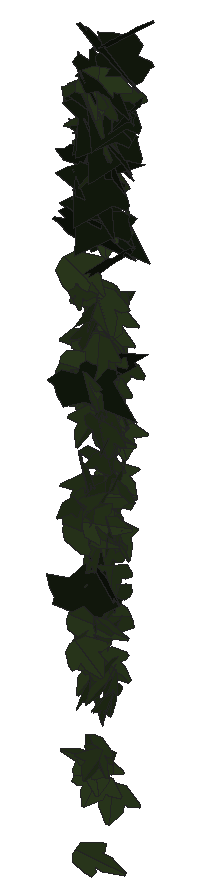
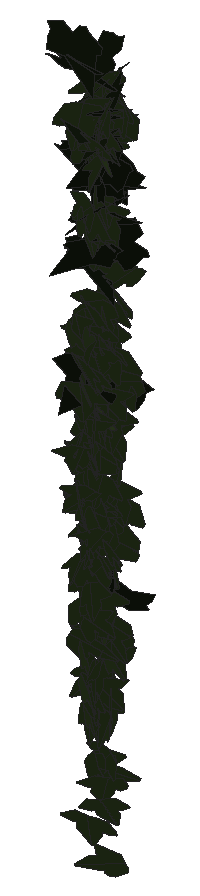
# SketchUp Ruby script. Lengths in inches.
U = 1.inch
M = Sketchup.active_model
def pt(a) = Geom::Point3d.new(a.map { |v| v * U })
def face(e, loops, mat)
  f = e.add_face(loops[0].map { |a| pt(a) })
  loops[1..].each { |l| e.add_face(l.map { |a| pt(a) }).erase! }
  f.material = f.back_material = mat if mat
  f
end
# faces: each face lists its corners as indices into pts; further lists are holes
def faces(e, pts, list, mat = nil) = list.each { |f| face(e, (f[0].is_a?(Array) ? f : [f]).map { |l| l.map { |i| pts[i] } }, mat) }
# xy, xz, yz: faces in a plane at the given z, y or x. An outline is a flat list of corners, or four numbers for a rectangle; further outlines are holes
def ring(l) = l.size == 4 ? [[l[0], l[1]], [l[2], l[1]], [l[2], l[3]], [l[0], l[3]]] : l.each_slice(2).to_a
def flat(e, list, mat, &to3) = list.each { |f| face(e, (f[0].is_a?(Array) ? f : [f]).map { |l| ring(l).map { |u, v| to3.(u, v) } }, mat) }
def xy(e, z, list, mat = nil) = flat(e, list, mat) { |x, y| [x, y, z] }
def xz(e, y, list, mat = nil) = flat(e, list, mat) { |x, z| [x, y, z] }
def yz(e, x, list, mat = nil) = flat(e, list, mat) { |y, z| [x, y, z] }
def lines(e, pts, list) = list.each { |a, b| e.add_line(pt(pts[a]), pt(pts[b])) }
# prism: a flat outline (further loops are holes) pulled along v
def prism(e, loops, v, mat = nil)
  f = face(e, loops, mat); d = Geom::Vector3d.new(v.map { |x| x * U })
  f.pushpull(f.normal.samedirection?(d) ? d.length : -d.length)
end
def box(e, o, s, mat = nil) = prism(e, [[o, [o[0] + s[0], o[1], o[2]], [o[0] + s[0], o[1] + s[1], o[2]], [o[0], o[1] + s[1], o[2]]]], [0, 0, s[2]], mat)
def at(x, y, z, deg = 0) = Geom::Transformation.translation(pt([x, y, z])) * Geom::Transformation.rotation(ORIGIN, Z_AXIS, deg.degrees)
def axes(o, x, y, z) = Geom::Transformation.new([*x, 0, *y, 0, *z, 0, *pt(o).to_a, 1])
def part(name) = M.definitions.add(name)
# library, detail: a bought-in or finely detailed component or shape, given as its bounding box
def library(name, o, s) = part(name).tap { |d| box(d.entities, o, s) }
def detail(e, o, s) = box(e.add_group.entities, o, s)
def put(e, d, t, mat = nil) = e.add_instance(d, t).tap { |i| i.material = mat if mat }
def group(e, t, mat = nil) = e.add_group.tap { |g| g.transformation = t; g.material = mat if mat }.entities
root = M.entities
M.materials.add("1026 AP 7946 SUNNY SIDE UP").color = [254, 231, 186]
M.materials.add("efeu1").color = [18, 25, 13]
M.materials.add("efeu2").color = [43, 57, 29]
c1 = part("ivyleaf_9")
p = [[1.54,2.16,1.25],[1.36,2.04,1.19],[-0.21,0.99,0.68],[-0.71,1.11,0.82],[-0.85,0.86,0.67],[-0.8,0.17,0.21],
  [-0.9,-0.01,0.1],[-0.67,-0.16,-0.02],[-0.08,-0.08,-0.05],[-0.03,-0.6,-0.4],[0.65,-0.88,-0.66],[0.83,-0.6,-0.49],
  [1.29,-0.42,-0.43],[1.8125,-0.07,-0.26],[1.21,0.44,0.15]]
faces(c1.entities,p,[[0,1,2,3,4,5,6,7,8,9,10,11,12,13,14]],"efeu1")
c2 = part("ivyleaf_10")
p = [[0,0.5,-0.03],[-0.0625,2.02,-0.43],[-0.19,2.01,-0.46],[-0.54,1.05,-0.29],[-0.52,0.625,-0.18],[-0.83,0.76,-0.28],
  [-1.16,0.64,-0.33],[-1.15,0.33,-0.24],[-0.77,-0.39,0.02],[-0.3,-0.51,0.16],[0.04,-0.48,0.23],[-0.02,2.01,-0.4375],
  [-0.06,2.01,-0.43],[0.04,-0.49,0.23],[0.67,-0.49,0.14],[1.38,0.36,-0.2],[1.375,0.51,-0.24],[0.81,0.65,-0.19],
  [0.62,0.59,-0.15],[0.6,1.09,-0.28],[0.5,1.23,-0.31]]
faces(c2.entities,p,[[0,1,2,3,4,5,6,7,8,9,10],[11,12,0,13,14,15,16,17,18,19,20]],"efeu2")
put(root,c1,axes([99.98,212.74,266.96],[0.2561,-0.12332,-0.15001],[-0.19651,0.07688,-0.20719],[0.24595,0.18983,-0.00934]),"1026 AP 7946 SUNNY SIDE UP")
put(root,c2,axes([100.08,212.81,261.875],[-0.07144,-0.19409,0.10989],[0.01651,-0.11176,-0.20345],[0.34869,-0.03448,0.03215]),"1026 AP 7946 SUNNY SIDE UP")
put(root,c2,axes([100.01,212.55,260.71],[-0.11557,-0.16973,-0.13356],[0.10562,0.11071,-0.18931],[0.31782,-0.09851,0.01435]),"1026 AP 7946 SUNNY SIDE UP")
put(root,c2,axes([100.11,212.6875,260.96],[-0.13002,-0.19505,0.05375],[-0.0144,-0.05389,-0.2182],[0.31761,-0.08229,0.01211]),"1026 AP 7946 SUNNY SIDE UP")
put(root,c2,axes([100.03,212.85,266.73],[-0.11221,0.20115,0.01139],[-0.01441,0.00565,-0.22649],[-0.34142,-0.06635,0.00581]),"1026 AP 7946 SUNNY SIDE UP")
put(root,c2,axes([100.05,212.87,257.73],[-0.19778,0.15965,-0.00779],[-0.00601,-0.01377,-0.20912],[-0.25131,-0.12531,0.01113]),"1026 AP 7946 SUNNY SIDE UP")
put(root,c2,axes([100.09,212.73,258.65],[-0.00028,-0.1767,0.06695],[0.00209,-0.06484,-0.19007],[0.3195,0.00027,0.0013]),"1026 AP 7946 SUNNY SIDE UP")
put(root,c2,axes([100.03,212.95,266],[-0.02915,0.2403,0.06293],[-0.01382,0.05921,-0.24791],[-0.3891,-0.02011,0.00409]),"1026 AP 7946 SUNNY SIDE UP")
put(root,c2,axes([100.11,212.93,265.09],[-0.09304,-0.21967,0.08481],[-0.00156,-0.08595,-0.23395],[0.36956,-0.05566,0.02037]),"1026 AP 7946 SUNNY SIDE UP")
put(root,c2,axes([100.1,212.66,257.96],[0.04722,-0.18143,-0.13844],[-0.00364,0.13428,-0.18796],[0.35404,0.02558,0.01653]),"1026 AP 7946 SUNNY SIDE UP")
put(root,c2,axes([100.28,213.01,262.125],[-0.10031,0.05849,-0.17741],[-0.24494,0.08504,0.088],[0.17242,0.15484,0.02181]),"1026 AP 7946 SUNNY SIDE UP")
put(root,c2,axes([100.15,212.87,262.39],[-0.18592,-0.14037,0.13697],[-0.04835,-0.1411,-0.18138],[0.30101,-0.10936,0.05546]),"1026 AP 7946 SUNNY SIDE UP")
put(root,c2,axes([100.12,212.81,262.14],[-0.17943,-0.19917,0.01326],[-0.00238,-0.01526,-0.23648],[0.31394,-0.11395,0.00578]),"1026 AP 7946 SUNNY SIDE UP")
put(root,c2,axes([100.13,213.07,259.23],[-0.0676,-0.11247,0.14072],[-0.02657,-0.13348,-0.12781],[0.29437,-0.03788,0.02078]),"1026 AP 7946 SUNNY SIDE UP")
put(root,c1,axes([99.88,212.88,265.98],[0.37658,-0.06604,-0.00176],[-0.01103,-0.02042,-0.25509],[0.10328,0.23863,-0.0208]),"1026 AP 7946 SUNNY SIDE UP")
put(root,c2,axes([100.24,212.68,258.88],[-0.23707,-0.00449,0.11586],[-0.17938,-0.03359,-0.14786],[0.04086,-0.1735,0.02311]),"1026 AP 7946 SUNNY SIDE UP")
put(root,c2,axes([100.13,212.84,258.15],[-0.10774,-0.1442,0.13203],[-0.0042,-0.13612,-0.15903],[0.30418,-0.05296,0.04457]),"1026 AP 7946 SUNNY SIDE UP")
put(root,c2,axes([100.05,212.94,260.39],[0.24772,-0.11603,0.05224],[0.04602,-0.04632,-0.19923],[0.20969,0.14724,-0.01798]),"1026 AP 7946 SUNNY SIDE UP")
put(root,c2,axes([99.93,212.79,266.61],[-0.27223,-0.04151,-0.1575],[0.25077,0.00963,-0.17582],[0.0632,-0.21705,0.01917]),"1026 AP 7946 SUNNY SIDE UP")
put(root,c1,axes([99.8125,212.66,264.71],[0.34732,-0.01776,0.10355],[0.15933,-0.03311,-0.219],[0.05109,0.22398,-0.02095]),"1026 AP 7946 SUNNY SIDE UP")
put(root,c2,axes([99.9,212.7,263.78],[0.01136,-0.08409,-0.19453],[0.20742,-0.141,0.07316],[-0.26711,-0.11306,0.04854]),"1026 AP 7946 SUNNY SIDE UP")
put(root,c2,axes([100.15,212.91,259.5],[-0.18067,-0.17133,0.04088],[-0.01251,-0.04344,-0.21203],[0.2766,-0.11388,0.01711]),"1026 AP 7946 SUNNY SIDE UP")
put(root,c2,axes([100.32,212.69,256.89],[0.01873,-0.00477,-0.19304],[-0.30598,0.00462,-0.01188],[0.00833,0.18053,-0.00227]),"1026 AP 7946 SUNNY SIDE UP")
put(root,c2,axes([100.09,212.77,263.02],[-0.34476,-0.07751,-0.0319],[0.06762,-0.02482,-0.22966],[0.123,-0.20361,0.03685]),"1026 AP 7946 SUNNY SIDE UP")
put(root,c2,axes([100.16,212.78,262.24],[-0.20673,0.16376,0.05791],[-0.09877,0.02061,-0.21526],[-0.27441,-0.13079,0.03385]),"1026 AP 7946 SUNNY SIDE UP")
put(root,c2,axes([100.03,213.02,260.5],[0.07929,0.15347,0.10104],[0.03237,0.09066,-0.17031],[-0.30234,0.04995,0.00826]),"1026 AP 7946 SUNNY SIDE UP")
put(root,c2,axes([100.01,212.59,262.49],[-0.25506,0.06591,-0.0971],[0.13004,-0.05234,-0.17565],[-0.14059,-0.16799,0.01369]),"1026 AP 7946 SUNNY SIDE UP")
put(root,c2,axes([100.14,212.71,263.27],[-0.02037,-0.22162,-0.00804],[-0.00083,0.00465,-0.23754],[0.37628,-0.01199,-0.00096]),"1026 AP 7946 SUNNY SIDE UP")
put(root,c2,axes([100.17,212.68,266.67],[-0.37665,0.07613,0.02777],[-0.06008,-0.03399,-0.25518],[-0.11162,-0.23859,0.04365]),"1026 AP 7946 SUNNY SIDE UP")
put(root,c2,axes([100.15,212.91,262.07],[0.01552,-0.15142,-0.17887],[-0.01077,0.17266,-0.15529],[0.36108,0.01166,0.00306]),"1026 AP 7946 SUNNY SIDE UP")
put(root,c2,axes([99.88,212.61,262.625],[-0.05132,-0.04659,-0.21433],[0.32465,0.06613,-0.04662],[0.12509,-0.19073,0.03305]),"1026 AP 7946 SUNNY SIDE UP")
put(root,c2,axes([100.13,212.91,261.23],[-0.30889,0.0208,-0.00815],[0.01069,-0.01418,-0.19575],[-0.03623,-0.18158,0.01177]),"1026 AP 7946 SUNNY SIDE UP")
put(root,c2,axes([100.14,212.81,265.45],[-0.01108,-0.24529,-0.02923],[0.01998,0.0266,-0.25235],[0.38751,-0.00838,0.01217]),"1026 AP 7946 SUNNY SIDE UP")
put(root,c2,axes([99.89,213.05,261.67],[0.00411,-0.01543,-0.1916],[0.26809,-0.08469,0.00893],[-0.1446,-0.15746,0.01112]),"1026 AP 7946 SUNNY SIDE UP")
put(root,c2,axes([100.08,212.99,258.62],[-0.04096,0.19002,-0.07512],[0.00219,-0.07443,-0.19785],[-0.32064,-0.02478,0.00824]),"1026 AP 7946 SUNNY SIDE UP")
put(root,c2,axes([100.16,212.97,260.76],[-0.04196,-0.17177,0.04384],[-0.01248,-0.04258,-0.18638],[0.30041,-0.02576,-0.00162]),"1026 AP 7946 SUNNY SIDE UP")
put(root,c2,axes([99.98,212.52,264.16],[0.12602,0.16921,0.14142],[0.11229,0.11249,-0.19579],[-0.34427,0.09863,-0.0121]),"1026 AP 7946 SUNNY SIDE UP")
put(root,c2,axes([100.125,212.84,256.49],[0.25373,0.07747,-0.06071],[-0.06832,-0.04672,-0.17938],[-0.14908,0.15326,-0.02112]),"1026 AP 7946 SUNNY SIDE UP")
put(root,c2,axes([100.1,212.98,260.22],[0.20563,-0.13762,0.04758],[0.03076,-0.04542,-0.19617],[0.24452,0.12145,-0.01533]),"1026 AP 7946 SUNNY SIDE UP")
put(root,c2,axes([100.18,212.82,266.26],[-0.21238,-0.21279,0.02009],[0.00455,-0.02631,-0.25924],[0.33614,-0.13409,0.0162]),"1026 AP 7946 SUNNY SIDE UP")
put(root,c2,axes([100.14,213.06,259.68],[-0.05708,-0.17961,-0.01684],[0.03431,0.00977,-0.19453],[0.30381,-0.03485,0.0188]),"1026 AP 7946 SUNNY SIDE UP")
put(root,c2,axes([100.14,212.54,261.25],[-0.19747,0.15947,0.01842],[-0.03825,0.00222,-0.21052],[-0.26923,-0.11728,0.0164]),"1026 AP 7946 SUNNY SIDE UP")
put(root,c2,axes([100.08,212.9375,266.11],[0.14856,-0.17461,0.15388],[0.09261,-0.13881,-0.205],[0.35029,0.11075,-0.01106]),"1026 AP 7946 SUNNY SIDE UP")
put(root,c2,axes([100.14,213.03,260.08],[-0.17523,0.14165,0.04059],[0.04836,-0.02381,0.18707],[0.24337,0.10672,-0.00795]),"1026 AP 7946 SUNNY SIDE UP")
put(root,c2,axes([100.35,213.05,258.89],[-0.09816,-0.00004,0.18134],[-0.25833,-0.07858,-0.05674],[0.12625,-0.16081,0.0249]),"1026 AP 7946 SUNNY SIDE UP")
put(root,c2,axes([100.11,213.2,263.32],[-0.02996,0.03401,-0.18638],[-0.01943,-0.17525,-0.03777],[-0.30123,0.00792,0.02097]),"1026 AP 7946 SUNNY SIDE UP")
put(root,c2,axes([100.19,212.84,266.31],[0.29185,-0.15682,-0.06163],[-0.07276,0.03654,-0.2501],[0.25317,0.19128,-0.00084]),"1026 AP 7946 SUNNY SIDE UP")
put(root,c2,axes([100.18,212.67,263.57],[0.0302,-0.22951,-0.05344],[-0.00262,0.05061,-0.23696],[0.36953,0.01911,0.00269]),"1026 AP 7946 SUNNY SIDE UP")
put(root,c2,axes([100.18,212.96,260.83],[-0.18303,-0.14312,0.00848],[0.00909,-0.01625,-0.19148],[0.24335,-0.10704,0.01353]),"1026 AP 7946 SUNNY SIDE UP")
put(root,c2,axes([100.16,212.93,258.48],[-0.00445,-0.19795,-0.05921],[0.03032,0.05585,-0.2028],[0.32221,-0.00799,0.01826]),"1026 AP 7946 SUNNY SIDE UP")
put(root,c2,axes([100.03,212.71,266.62],[-0.26103,0.10636,-0.15853],[0.14847,-0.13087,-0.19811],[-0.25483,-0.1852,0.04697]),"1026 AP 7946 SUNNY SIDE UP")
put(root,c2,axes([100.01,212.87,262.1],[0.10307,-0.15186,-0.07926],[0.14061,-0.03963,0.16359],[-0.24829,-0.08549,0.05974]),"1026 AP 7946 SUNNY SIDE UP")
put(root,c2,axes([100.15,212.86,266.58],[-0.28719,0.17,-0.02382],[0.00822,-0.02965,-0.25655],[-0.26985,-0.18183,0.01754]),"1026 AP 7946 SUNNY SIDE UP")
put(root,c2,axes([100.09,212.87,260.28],[-0.09177,-0.14046,0.1231],[0.05218,0.11309,0.16239],[-0.3057,0.06147,-0.00924]),"1026 AP 7946 SUNNY SIDE UP")
put(root,c2,axes([100.15,212.9,260.41],[-0.03733,-0.17264,-0.13319],[0.07661,0.12141,-0.17688],[0.32943,-0.0478,0.02604]),"1026 AP 7946 SUNNY SIDE UP")
put(root,c2,axes([100.09,212.91,258.74],[-0.09936,0.0959,0.182],[0.15854,-0.14442,0.11744],[0.27257,0.11896,-0.00197]),"1026 AP 7946 SUNNY SIDE UP")
put(root,c2,axes([100.23,212.84,259.42],[-0.01481,-0.15875,0.08975],[-0.00752,-0.08579,-0.1714],[0.30631,-0.00978,0.00013]),"1026 AP 7946 SUNNY SIDE UP")
put(root,c1,axes([100.18,212.5,259.27],[-0.30069,-0.00675,0.15175],[0.23054,0.01764,0.19697],[-0.02532,0.24077,-0.00876]),"1026 AP 7946 SUNNY SIDE UP")
put(root,c2,axes([100.27,212.79,262.03],[-0.28947,0.11073,0.05305],[-0.09254,0.00367,-0.21585],[-0.18287,-0.17714,0.02526]),"1026 AP 7946 SUNNY SIDE UP")
put(root,c2,axes([100.26,212.9,263.64],[-0.20074,-0.18705,0.06779],[-0.01402,-0.07401,-0.23125],[0.31204,-0.12366,0.03323]),"1026 AP 7946 SUNNY SIDE UP")
put(root,c2,axes([100.13,212.9375,264.66],[0.20547,0.16464,-0.0052],[0.0091,-0.01262,-0.21858],[-0.27958,0.12059,-0.01094]),"1026 AP 7946 SUNNY SIDE UP")
put(root,c2,axes([99.91,212.61,260.22],[-0.03407,0.0179,0.24638],[0.37307,0.03592,0.01959],[-0.0539,0.23733,-0.02012]),"1026 AP 7946 SUNNY SIDE UP")
put(root,c2,axes([100.26,212.93,259.93],[-0.16614,-0.16265,0.09748],[-0.01623,-0.10436,-0.19539],[0.29617,-0.09696,0.04397]),"1026 AP 7946 SUNNY SIDE UP")
put(root,c2,axes([100.23,212.63,260.04],[0.21488,-0.16875,-0.04831],[-0.03091,0.0431,-0.22313],[0.27326,0.13758,0.01275]),"1026 AP 7946 SUNNY SIDE UP")
put(root,c2,axes([100.24,212.89,261.9],[0.19349,-0.15581,-0.11371],[-0.04241,0.11479,-0.19883],[0.29642,0.11813,0.04578]),"1026 AP 7946 SUNNY SIDE UP")
put(root,c2,axes([100.1,212.81,263],[-0.29027,0.07828,-0.11866],[0.1506,-0.06848,-0.20569],[-0.15976,-0.20678,0.02169]),"1026 AP 7946 SUNNY SIDE UP")
put(root,c2,axes([100.13,212.76,256.77],[0.22233,0.13184,0.00986],[0.02547,-0.00438,-0.19847],[-0.22272,0.13111,-0.01286]),"1026 AP 7946 SUNNY SIDE UP")
put(root,c2,axes([100.25,213,265.08],[-0.02626,-0.23827,-0.03461],[-0.00083,0.03236,-0.24586],[0.37806,-0.01648,-0.00294]),"1026 AP 7946 SUNNY SIDE UP")
put(root,c2,axes([100.18,212.95,263.1],[0.30717,0.06464,-0.01952],[-0.01933,-0.02455,-0.20502],[-0.11276,0.18029,-0.01803]),"1026 AP 7946 SUNNY SIDE UP")
put(root,c2,axes([100.24,212.75,260.71],[-0.02305,-0.1831,0.12605],[0.02243,-0.1242,-0.18883],[0.34647,-0.00414,0.02061]),"1026 AP 7946 SUNNY SIDE UP")
put(root,c1,axes([100.0625,212.79,267.06],[0.18374,-0.20461,-0.10331],[-0.04706,0.09663,-0.24128],[0.35438,0.11892,0.02152]),"1026 AP 7946 SUNNY SIDE UP")
put(root,c1,axes([100.08,212.8125,265.3],[0.07966,-0.22509,-0.00624],[-0.01257,0.00142,-0.24602],[0.38192,0.04699,-0.00679]),"1026 AP 7946 SUNNY SIDE UP")
put(root,c2,axes([100.37,212.88,260.84],[-0.29247,-0.01327,0.0929],[-0.1365,-0.05372,-0.18011],[0.06049,-0.18536,0.04273]),"1026 AP 7946 SUNNY SIDE UP")
put(root,c2,axes([100.27,212.98,263.5625],[-0.11157,-0.22048,0.01853],[0.00906,-0.02204,-0.2384],[0.34788,-0.07014,0.01215]),"1026 AP 7946 SUNNY SIDE UP")
put(root,c2,axes([100.22,213.05,266.22],[0.31913,-0.08345,-0.00431],[-0.01691,-0.01523,-0.21957],[0.14074,0.1874,-0.01661]),"1026 AP 7946 SUNNY SIDE UP")
put(root,c2,axes([100.28,212.83,266.21],[-0.23585,0.19054,0.0542],[-0.07923,0.02561,-0.24851],[-0.30008,-0.15652,0.02302]),"1026 AP 7946 SUNNY SIDE UP")
put(root,c1,axes([99.95,212.74,265.55],[0.05368,-0.03107,0.22719],[0.35217,-0.05154,-0.04181],[0.09497,0.20868,0.02665]),"1026 AP 7946 SUNNY SIDE UP")
put(root,c2,axes([100.27,213.1,262.96],[0.23399,-0.11743,-0.03457],[-0.05608,0.00849,-0.1931],[0.19829,0.14098,-0.01382]),"1026 AP 7946 SUNNY SIDE UP")
put(root,c2,axes([100.14,212.49,258.58],[0.13212,0.16649,0.11102],[0.04791,0.09855,-0.19479],[-0.32754,0.08157,0.01629]),"1026 AP 7946 SUNNY SIDE UP")
put(root,c2,axes([100.3,213.11,262.57],[-0.29941,-0.04436,0.02868],[-0.03708,-0.02478,-0.19404],[0.08033,-0.17676,0.01733]),"1026 AP 7946 SUNNY SIDE UP")
put(root,c2,axes([100.28,212.87,258.02],[-0.01429,-0.13224,0.15764],[0.00503,-0.154,-0.13715],[0.31887,-0.0035,0.00923]),"1026 AP 7946 SUNNY SIDE UP")
put(root,c2,axes([100.32,212.68,256.99],[-0.11387,-0.16038,0.08274],[-0.03734,-0.07674,-0.18696],[0.30148,-0.07008,0.0081]),"1026 AP 7946 SUNNY SIDE UP")
put(root,c1,axes([100.01,212.86,267.42],[0.25982,-0.18693,0.04306],[0.05346,-0.02713,-0.25707],[0.29679,0.16854,0.00861]),"1026 AP 7946 SUNNY SIDE UP")
put(root,c1,axes([100.33,212.88,266.42],[-0.30027,-0.15691,0.03409],[-0.02887,-0.03111,-0.25449],[0.25079,-0.19145,0.01152]),"1026 AP 7946 SUNNY SIDE UP")
put(root,c2,axes([100.25,212.78,260.53],[0.0318,-0.18886,0.10968],[0.05208,-0.10406,-0.1953],[0.33775,0.03383,0.01979]),"1026 AP 7946 SUNNY SIDE UP")
put(root,c1,axes([100.05,212.89,266.25],[0.18139,-0.22132,0.0105],[0.02599,-0.00427,-0.25681],[0.3475,0.11585,0.01373]),"1026 AP 7946 SUNNY SIDE UP")
put(root,c1,axes([100.32,212.78,264.96],[-0.29808,-0.14089,0.00623],[0.00974,-0.01935,-0.24046],[0.23932,-0.17469,0.01755]),"1026 AP 7946 SUNNY SIDE UP")
put(root,c2,axes([100.08,212.84,265.94],[-0.0261,0.01416,-0.22561],[0.18922,-0.17915,-0.02407],[-0.30491,-0.11238,0.00437]),"1026 AP 7946 SUNNY SIDE UP")
put(root,c2,axes([100.19,212.71,257.11],[-0.22695,0.08535,-0.10662],[0.09298,-0.09453,-0.16496],[-0.20389,-0.13812,0.04345]),"1026 AP 7946 SUNNY SIDE UP")
put(root,c1,axes([100.3,212.73,265.43],[-0.28014,-0.15877,0.00838],[0.00625,-0.01806,-0.24485],[0.26996,-0.16433,0.01436]),"1026 AP 7946 SUNNY SIDE UP")
put(root,c2,axes([100.29,213,258.76],[0.02621,-0.20305,-0.00064],[0.00597,-0.00022,-0.20985],[0.31921,0.01668,0.00398]),"1026 AP 7946 SUNNY SIDE UP")
put(root,c2,axes([100.26,212.93,263.6875],[0.2591,-0.1186,0.01456],[0.00408,-0.02152,-0.20657],[0.20292,0.15186,-0.01444]),"1026 AP 7946 SUNNY SIDE UP")
put(root,c2,axes([100.3125,213.19,263.52],[-0.01301,-0.17252,0.0651],[-0.00712,-0.06293,-0.18575],[0.31173,-0.00864,-0.00152]),"1026 AP 7946 SUNNY SIDE UP")
put(root,c1,axes([100.08,212.54,262.56],[-0.02507,-0.08114,-0.24842],[0.13524,0.22518,-0.08276],[0.37577,-0.08645,0.01321]),"1026 AP 7946 SUNNY SIDE UP")
put(root,c1,axes([100.13,212.97,264.66],[0.02274,-0.10114,-0.20309],[0.03867,0.18835,-0.1039],[0.36089,-0.01381,0.02393]),"1026 AP 7946 SUNNY SIDE UP")
put(root,c2,axes([100.3,212.76,260.9375],[-0.0679,-0.20815,-0.0608],[0.02276,0.05606,-0.21865],[0.33893,-0.04547,0.0025]),"1026 AP 7946 SUNNY SIDE UP")
put(root,c2,axes([100.1875,213.11,265.28],[-0.1892,0.1121,-0.12441],[0.10793,-0.10123,-0.16913],[-0.25389,-0.12657,0.02081]),"1026 AP 7946 SUNNY SIDE UP")
put(root,c1,axes([100.12,212.81,265.17],[0.12169,-0.20764,-0.11247],[-0.00635,0.11254,-0.22524],[0.36796,0.07062,0.03331]),"1026 AP 7946 SUNNY SIDE UP")
put(root,c2,axes([100.21,213.01,256.29],[0.32473,0.03645,0.01744],[0.03115,-0.01642,-0.2152],[-0.05482,0.20654,-0.01893]),"1026 AP 7946 SUNNY SIDE UP")
put(root,c2,axes([100.25,212.96,262.82],[0.29733,-0.07608,0.02008],[0.01825,-0.0246,-0.20385],[0.13217,0.17454,-0.01703]),"1026 AP 7946 SUNNY SIDE UP")
put(root,c2,axes([100.02,212.62,258.91],[0.05312,0.02238,0.22947],[0.30553,0.10869,-0.041],[-0.17442,0.1972,-0.00193]),"1026 AP 7946 SUNNY SIDE UP")
put(root,c2,axes([100.22,212.73,263.72],[-0.35177,-0.02151,-0.08027],[0.1292,-0.09935,-0.19681],[-0.0268,-0.1966,0.10476]),"1026 AP 7946 SUNNY SIDE UP")
put(root,c2,axes([100.3125,212.96,258.25],[0.02992,-0.20216,0.02445],[0.00056,-0.02496,-0.20932],[0.32027,0.01893,-0.00192]),"1026 AP 7946 SUNNY SIDE UP")
put(root,c2,axes([100.28,212.91,258.09],[0.233,-0.14023,-0.02575],[0.00313,0.03698,-0.20796],[0.22374,0.14552,0.02973]),"1026 AP 7946 SUNNY SIDE UP")
put(root,c2,axes([100.21,212.71,263.02],[0.35581,-0.05175,0.0401],[0.06501,-0.00393,-0.23112],[0.08764,0.213,0.00863]),"1026 AP 7946 SUNNY SIDE UP")
put(root,c2,axes([100.29,212.99,262.61],[0.10153,-0.16731,0.05682],[0.02262,-0.05389,-0.19089],[0.29825,0.06104,-0.00487]),"1026 AP 7946 SUNNY SIDE UP")
put(root,c2,axes([100.33,212.8,266.02],[-0.20928,-0.2008,0.06095],[0.02261,-0.08001,-0.24221],[0.3289,-0.12227,0.05544]),"1026 AP 7946 SUNNY SIDE UP")
put(root,c1,axes([100.52,212.94,266.4],[-0.25901,0.18285,-0.04628],[-0.02511,-0.07435,-0.24617],[-0.2954,-0.15401,0.06151]),"1026 AP 7946 SUNNY SIDE UP")
put(root,c2,axes([100.34,212.99,260.3],[0.17022,-0.14908,-0.05768],[-0.03853,0.04728,-0.19153],[0.2652,0.10255,0.0092]),"1026 AP 7946 SUNNY SIDE UP")
put(root,c1,axes([100.32,212.81,266.36],[-0.23583,-0.18236,0.08163],[-0.01029,-0.09591,-0.23762],[0.31312,-0.1405,0.05367]),"1026 AP 7946 SUNNY SIDE UP")
put(root,c2,axes([100.25,212.72,266.9375],[0.19699,0.21431,-0.04714],[-0.01917,-0.04721,-0.25566],[-0.34445,0.12519,-0.01273]),"1026 AP 7946 SUNNY SIDE UP")
put(root,c2,axes([100.24,212.93,263.39],[0.30236,0.07454,0.00203],[0.01324,-0.01625,-0.20604],[-0.12584,0.17737,-0.0168]),"1026 AP 7946 SUNNY SIDE UP")
put(root,c2,axes([100.36,212.95,259.32],[-0.12164,-0.19206,0.03875],[-0.00806,-0.03962,-0.2133],[0.30797,-0.07689,0.00973]),"1026 AP 7946 SUNNY SIDE UP")
put(root,c2,axes([100.33,212.86,257.8],[-0.04525,-0.19676,-0.06127],[0.01301,0.05777,-0.20452],[0.32244,-0.02994,-0.00034]),"1026 AP 7946 SUNNY SIDE UP")
put(root,c1,axes([100.06,212.99,265.71],[0.0804,-0.04618,-0.24173],[0.36358,-0.05065,0.06195],[-0.09437,-0.23448,0.03274]),"1026 AP 7946 SUNNY SIDE UP")
put(root,c2,axes([100.35,212.89,260.92],[-0.31005,0.07275,0.01488],[-0.03061,-0.01039,-0.2099],[-0.12165,-0.18281,0.01489]),"1026 AP 7946 SUNNY SIDE UP")
put(root,c2,axes([100.34,213.04,261.98],[-0.16868,0.15037,0.05088],[-0.0581,0.0319,-0.19218],[-0.26032,-0.10456,0.00992]),"1026 AP 7946 SUNNY SIDE UP")
put(root,c2,axes([100.09,212.94,261.52],[-0.06749,0.01677,0.1855],[0.29364,0.02172,0.04059],[-0.02977,0.17623,-0.02014]),"1026 AP 7946 SUNNY SIDE UP")
put(root,c2,axes([100.32,212.77,261.41],[-0.10713,-0.20023,-0.07602],[0.05269,0.06525,-0.21726],[0.33075,-0.07525,0.00999]),"1026 AP 7946 SUNNY SIDE UP")
put(root,c2,axes([100.34,212.82,257.79],[0.02492,-0.20484,-0.00799],[0.00462,0.00684,-0.21158],[0.32222,0.01575,0.00365]),"1026 AP 7946 SUNNY SIDE UP")
put(root,c2,axes([100.32,212.64,262.34],[0.08475,0.02202,-0.22142],[0.04603,0.21047,0.03389],[0.35055,-0.03296,0.04908]),"1026 AP 7946 SUNNY SIDE UP")
put(root,c2,axes([100.33,213.02,266.57],[-0.24652,-0.18728,-0.04572],[0.08158,0.01259,-0.24948],[0.29103,-0.16217,0.03121]),"1026 AP 7946 SUNNY SIDE UP")
put(root,c2,axes([100.3125,212.875,261.8],[0.04771,0.2015,0.04271],[-0.03722,0.04036,-0.21534],[-0.34586,0.02345,0.02906]),"1026 AP 7946 SUNNY SIDE UP")
put(root,c2,axes([100.36,212.9,261.59],[0.17551,-0.17659,-0.00981],[-0.02298,0.00001,-0.21872],[0.29911,0.10362,-0.01105]),"1026 AP 7946 SUNNY SIDE UP")
put(root,c1,axes([100.32,212.9375,266.5],[-0.21052,-0.20651,0.04974],[0.01342,-0.06365,-0.25038],[0.33363,-0.12775,0.04146]),"1026 AP 7946 SUNNY SIDE UP")
put(root,c2,axes([100.25,212.81,258.34],[-0.17142,-0.12771,-0.12162],[0.16796,0.05973,-0.16887],[0.21482,-0.14861,0.03499]),"1026 AP 7946 SUNNY SIDE UP")
put(root,c2,axes([100.14,212.58,255.5],[0.07286,0.05101,0.18108],[0.22952,0.10149,-0.06836],[-0.19135,0.14116,-0.01304]),"1026 AP 7946 SUNNY SIDE UP")
put(root,c2,axes([100.375,212.83,259.67],[-0.19086,-0.15443,-0.00366],[0.01992,-0.00681,-0.20409],[0.26141,-0.11224,0.01288]),"1026 AP 7946 SUNNY SIDE UP")
put(root,c2,axes([100.375,213,261.04],[0.07771,-0.20671,-0.05043],[0.00088,0.04918,-0.21834],[0.3336,0.04802,0.01232]),"1026 AP 7946 SUNNY SIDE UP")
put(root,c1,axes([100.28,212.8,262.71],[0.21761,0.18492,0.07401],[0.08634,0.04714,-0.23717],[-0.29914,0.14813,-0.01461]),"1026 AP 7946 SUNNY SIDE UP")
put(root,c2,axes([100.33,213.06,260.1],[0.00881,0.18071,0.03826],[-0.01898,0.03364,-0.19265],[-0.31137,0.00306,0.01283]),"1026 AP 7946 SUNNY SIDE UP")
put(root,c1,axes([100.34,212.58,259.76],[0.2894,-0.06707,-0.14966],[-0.22696,0.02463,-0.20048],[0.10732,0.23294,-0.0204]),"1026 AP 7946 SUNNY SIDE UP")
put(root,c2,axes([100.4,212.77,261.75],[0.11082,-0.22024,-0.04564],[-0.02321,0.04048,-0.23798],[0.3521,0.07199,-0.00132]),"1026 AP 7946 SUNNY SIDE UP")
put(root,c2,axes([100.12,212.81,260.68],[0.12109,-0.04066,-0.18218],[0.29579,0.00777,0.07655],[-0.01427,-0.18387,0.04083]),"1026 AP 7946 SUNNY SIDE UP")
put(root,c2,axes([100.29,213.05,261.65],[0.22566,0.12566,0.0324],[0.04749,0.01201,-0.19535],[-0.21356,0.13545,-0.00921]),"1026 AP 7946 SUNNY SIDE UP")
put(root,c1,axes([100.39,212.88,266.09],[-0.23099,-0.19817,0.0329],[-0.00714,-0.03767,-0.25362],[0.31582,-0.14579,0.01833]),"1026 AP 7946 SUNNY SIDE UP")
put(root,c2,axes([100.41,212.58,261.91],[-0.33151,0.06831,0.00291],[-0.01426,-0.01852,-0.22068],[-0.11512,-0.19442,0.01897]),"1026 AP 7946 SUNNY SIDE UP")
put(root,c1,axes([100.51,212.65,264.39],[-0.05563,0.216,-0.06495],[0.01406,-0.06295,-0.23476],[-0.38191,-0.03378,0.00082]),"1026 AP 7946 SUNNY SIDE UP")
put(root,c2,axes([100.24,212.98,261.01],[0.15625,0.11966,0.11201],[0.1222,0.0744,-0.16025],[-0.23863,0.11645,-0.00872]),"1026 AP 7946 SUNNY SIDE UP")
put(root,c2,axes([100.28,212.58,260.43],[0.01499,0.06057,0.219],[0.07751,0.20649,-0.06178],[-0.33828,0.05,-0.00445]),"1026 AP 7946 SUNNY SIDE UP")
put(root,c1,axes([100.59,213.03,267.25],[-0.37386,0.01122,0.03887],[-0.06311,-0.02377,-0.23486],[-0.01214,-0.22192,0.02398]),"1026 AP 7946 SUNNY SIDE UP")
put(root,c2,axes([100.4,212.72,260.29],[0.09153,-0.13167,-0.15177],[0.01297,0.14681,-0.14256],[0.32605,0.03112,0.04828]),"1026 AP 7946 SUNNY SIDE UP")
put(root,c2,axes([100.26,213.01,262.26],[0.26497,-0.05383,0.10121],[0.141,-0.04969,-0.17649],[0.12086,0.17597,-0.01599]),"1026 AP 7946 SUNNY SIDE UP")
put(root,c1,axes([100.53,212.9375,267.6],[-0.02082,0.25338,-0.02148],[-0.02111,-0.02298,-0.26109],[-0.39939,-0.01199,0.01492]),"1026 AP 7946 SUNNY SIDE UP")
